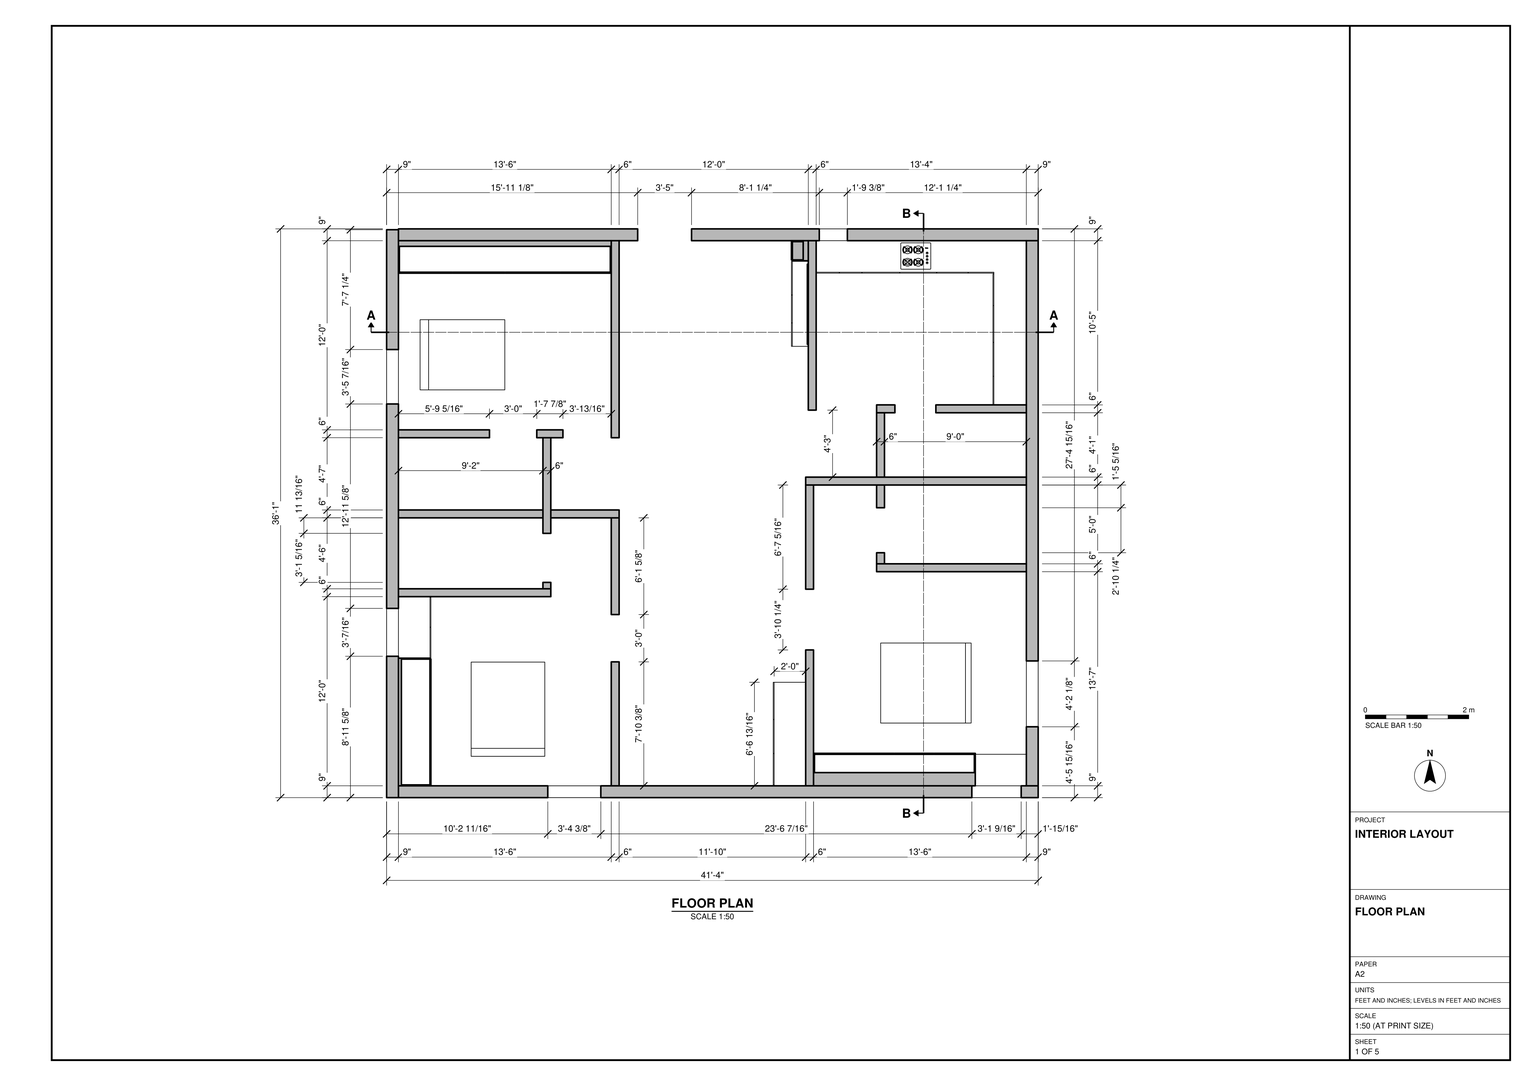
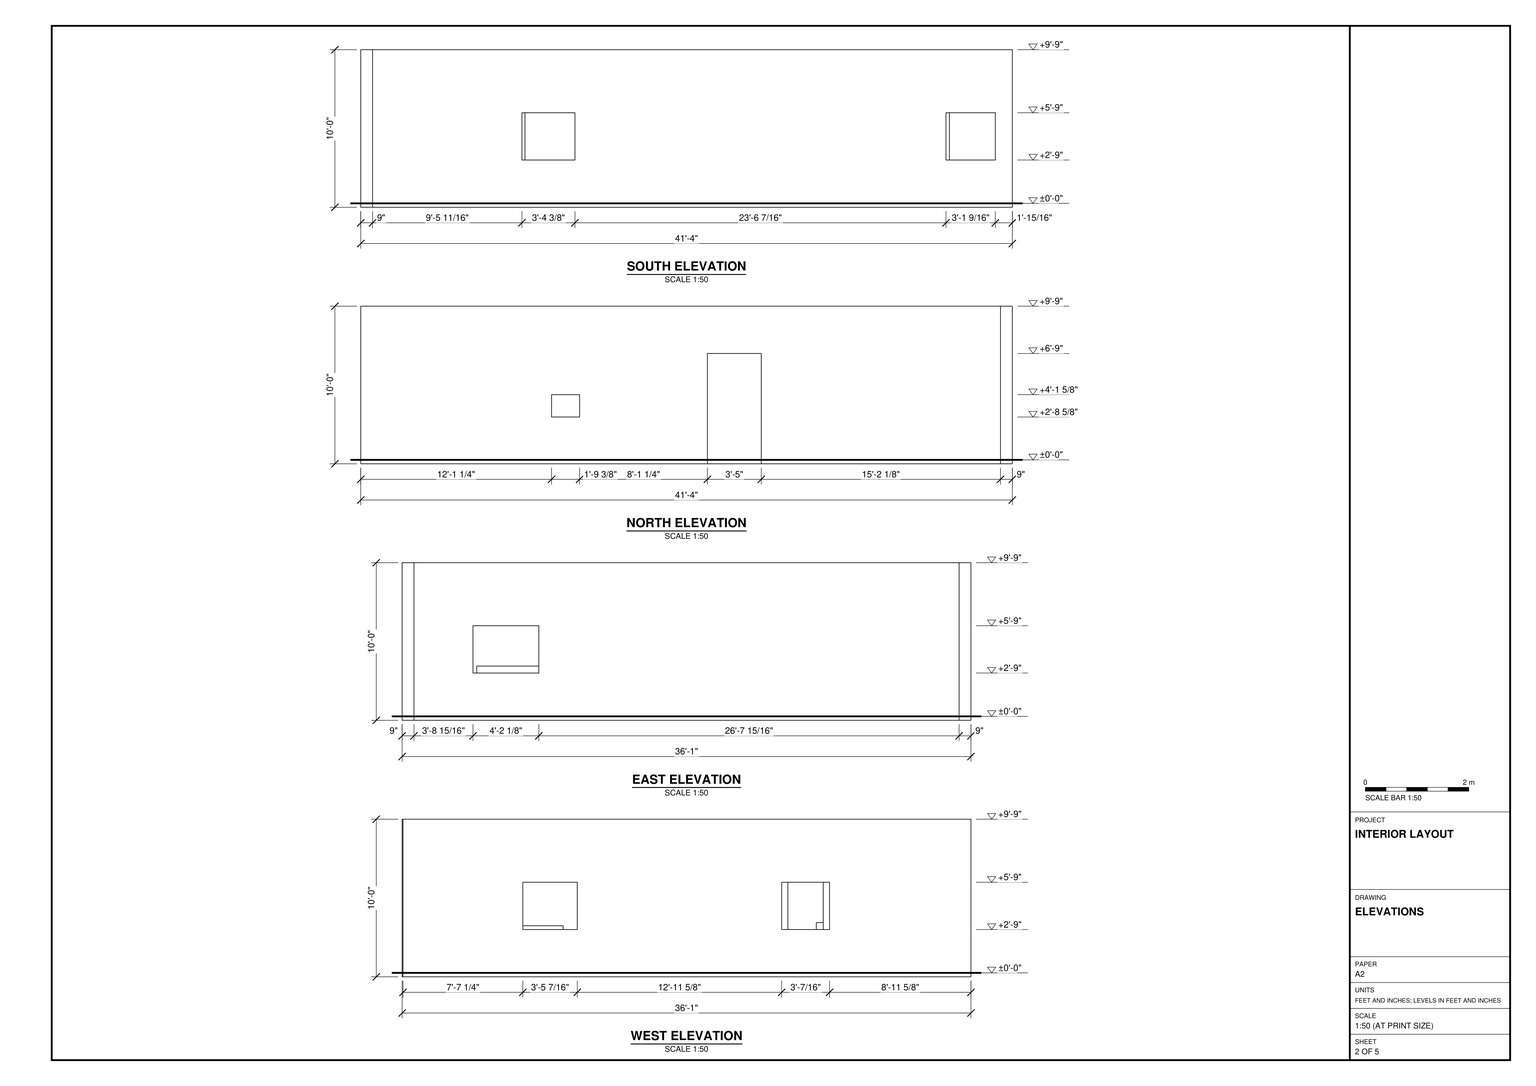
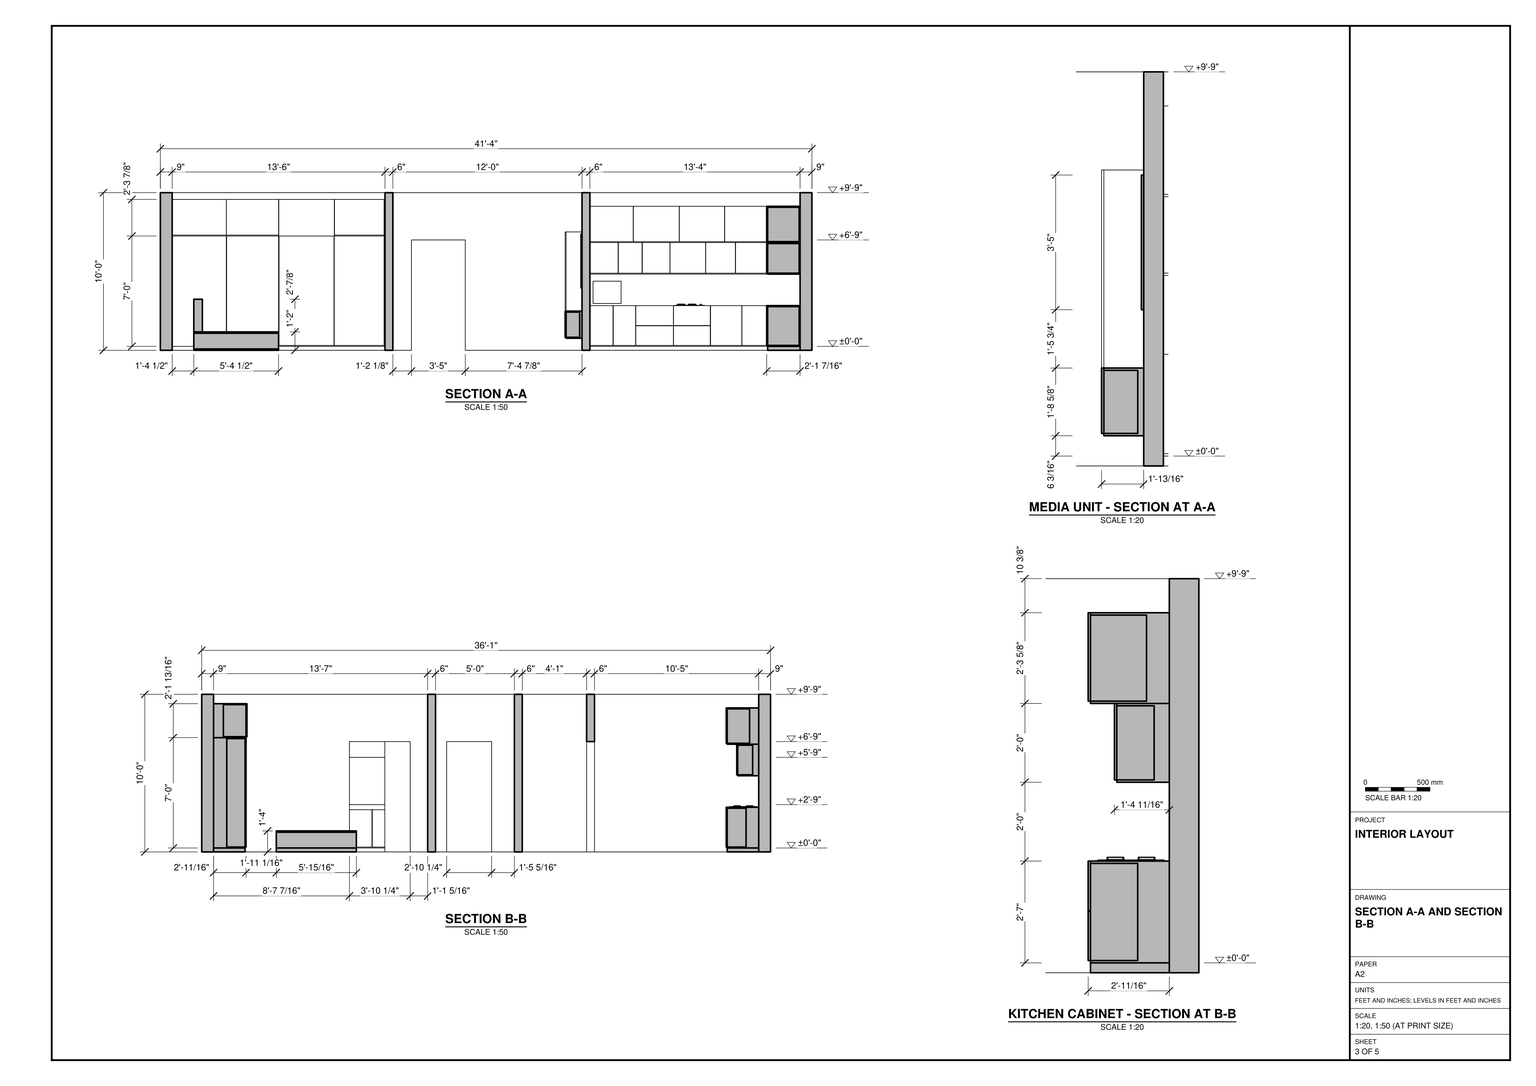
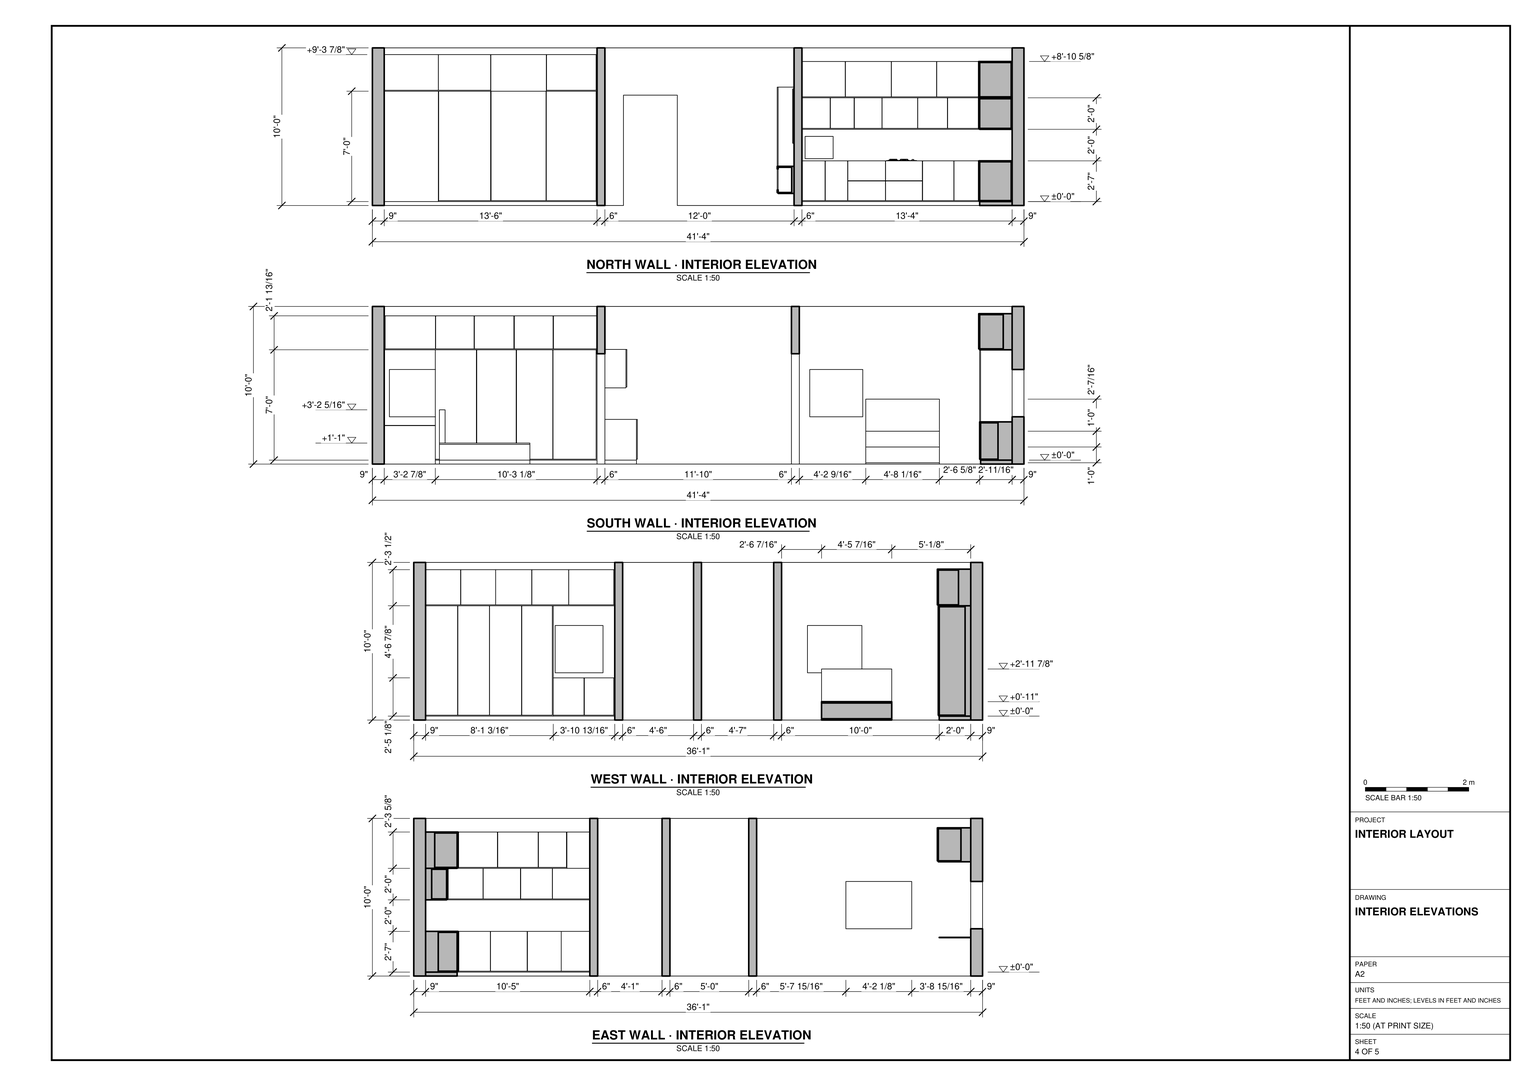
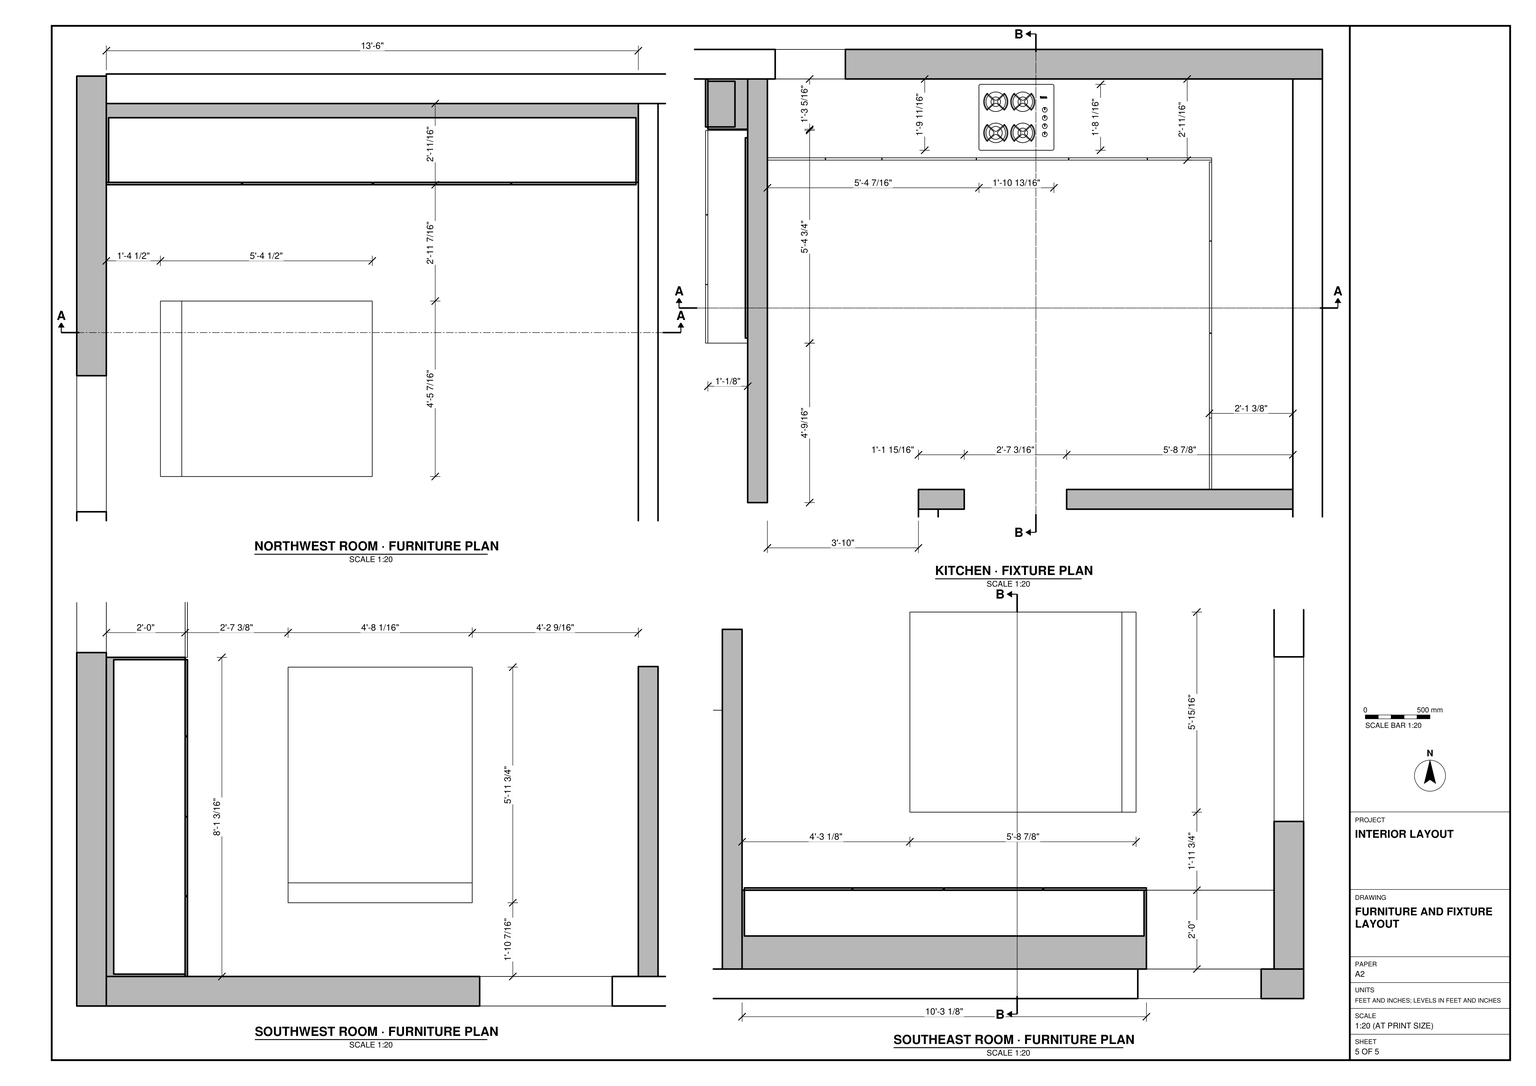
Build the single-storey interior in SketchUp from task_files/diagram_01.pdf. Work in feet and inches. Set the ground-floor datum at ±0'-0" and make the model 41'-4" east to west, 36'-1" north to south and 10'-0" high overall.

Lay out the 9" perimeter walls and 6" internal partitions from the floor plan. Keep the central circulation space open between the bedrooms and kitchen, and follow the partition returns and doorway gaps on either side. Use the elevations to distinguish the floor-level entrance on the north side from the raised window openings and to set the sills and heads.

Fit the northeast kitchen with a counter that turns along the east wall. Use the sections to set the depths and vertical arrangement of the cabinets, and place the cooktop on the north run. On the circulation side of the kitchen partition, model the media unit with its raised lower cabinet. Place the beds and wall storage in the northwest, southwest and southeast rooms, matching their footprints and orientations to the plan. Decor and loose items may be any suitable library components.

Keep shell elements such as walls and slabs separate, make each furniture or joinery piece a group or component, and use components for repeated parts. Save one SketchUp model as output_files/three_bedroom_interior_kitchen_and_built_in_storage.skp.

# SketchUp Ruby script. Lengths in inches.
U = 1.inch
M = Sketchup.active_model
def pt(a) = Geom::Point3d.new(a.map { |v| v * U })
def face(e, loops, mat)
  f = e.add_face(loops[0].map { |a| pt(a) })
  loops[1..].each { |l| e.add_face(l.map { |a| pt(a) }).erase! }
  f.material = f.back_material = mat if mat
  f
end
# faces: each face lists its corners as indices into pts; further lists are holes
def faces(e, pts, list, mat = nil) = list.each { |f| face(e, (f[0].is_a?(Array) ? f : [f]).map { |l| l.map { |i| pts[i] } }, mat) }
# xy, xz, yz: faces in a plane at the given z, y or x. An outline is a flat list of corners, or four numbers for a rectangle; further outlines are holes
def ring(l) = l.size == 4 ? [[l[0], l[1]], [l[2], l[1]], [l[2], l[3]], [l[0], l[3]]] : l.each_slice(2).to_a
def flat(e, list, mat, &to3) = list.each { |f| face(e, (f[0].is_a?(Array) ? f : [f]).map { |l| ring(l).map { |u, v| to3.(u, v) } }, mat) }
def xy(e, z, list, mat = nil) = flat(e, list, mat) { |x, y| [x, y, z] }
def xz(e, y, list, mat = nil) = flat(e, list, mat) { |x, z| [x, y, z] }
def yz(e, x, list, mat = nil) = flat(e, list, mat) { |y, z| [x, y, z] }
def lines(e, pts, list) = list.each { |a, b| e.add_line(pt(pts[a]), pt(pts[b])) }
# prism: a flat outline (further loops are holes) pulled along v
def prism(e, loops, v, mat = nil)
  f = face(e, loops, mat); d = Geom::Vector3d.new(v.map { |x| x * U })
  f.pushpull(f.normal.samedirection?(d) ? d.length : -d.length)
end
def box(e, o, s, mat = nil) = prism(e, [[o, [o[0] + s[0], o[1], o[2]], [o[0] + s[0], o[1] + s[1], o[2]], [o[0], o[1] + s[1], o[2]]]], [0, 0, s[2]], mat)
def at(x, y, z, deg = 0) = Geom::Transformation.translation(pt([x, y, z])) * Geom::Transformation.rotation(ORIGIN, Z_AXIS, deg.degrees)
def axes(o, x, y, z) = Geom::Transformation.new([*x, 0, *y, 0, *z, 0, *pt(o).to_a, 1])
def part(name) = M.definitions.add(name)
# library, detail: a bought-in or finely detailed component or shape, given as its bounding box
def library(name, o, s) = part(name).tap { |d| box(d.entities, o, s) }
def detail(e, o, s) = box(e.add_group.entities, o, s)
def put(e, d, t, mat = nil) = e.add_instance(d, t).tap { |i| i.material = mat if mat }
def group(e, t, mat = nil) = e.add_group.tap { |g| g.transformation = t; g.material = mat if mat }.entities
root = M.entities
c1 = library("1-TABLE DE CUISSON CLC2",[-11.42,-10.04,0],[22.84,20.08,1.26])
c2 = part("Group\#94")
box(c2.entities,[0,0,0],[8.25,13.9,0.71])
put(root,c1,at(402.83,412.33,34))
g1 = group(root,at(0,0,0))
prism(g1,[[[0,432.35,0],[0,0,0],[0,0,120],[0,432.35,120]],[[0,341.125,72],[0,299.6875,72],[0,299.6875,36],[0,341.125,36]],[[0,107.625,72],[0,107.625,36],[0,144.0625,36],[0,144.0625,72]]],[9,0,0])
g2 = group(root,at(9,0,0))
prism(g2,[[[0,0,0],[487,0,0],[487,0,120],[0,0,120]],[[113.6875,0,72],[154.0625,0,72],[154.0625,0,36],[113.6875,0,36]],[[436.5,0,72],[474.0625,0,72],[474.0625,0,36],[436.5,0,36]]],[0,9,0])
g3 = group(root,at(171,9,0))
prism(g3,[[[0,204,0],[0,130.375,0],[0,130.375,84],[0,94.375,84],[0,94.375,0],[0,0,0],[0,0,120],[0,204,120]]],[6,0,0])
g4 = group(root,at(9,153,0))
box(g4,[0,0,0],[116,6,120])
g5 = group(root,at(119,159,0))
xy(g5,0,[[0,0,6,4.875],[0,42.1875,6,115]])
xy(g5,84,[[0,4.875,6,42.1875]])
xy(g5,120,[[0,0,6,115]])
xz(g5,0,[[0,0,6,120]])
xz(g5,4.875,[[0,0,6,84]])
xz(g5,42.1875,[[0,0,6,84]])
xz(g5,115,[[0,0,6,120]])
yz(g5,0,[[0,0,0,120,54,120,54,0,42.1875,0,42.1875,84,4.875,84,4.875,0],[54,0,60,120],[60,0,115,120]])
yz(g5,6,[[0,0,4.875,0,4.875,84,42.1875,84,42.1875,0,54,0,54,120,0,120],[54,0,60,120],[60,0,115,120]])
g6 = group(root,at(9,274,0))
prism(g6,[[[69.3125,6,0],[0,6,0],[0,6,120],[162,6,120],[162,6,84],[125.22,6,84],[125.22,6,0],[105.3125,6,0],[105.3125,6,84],[69.3125,6,84]]],[0,-6,0])
g7 = group(root,at(171,274,0))
prism(g7,[[[0,150,0],[6,150,0],[6,0,0],[0,0,0],[0,141.51,0]]],[0,0,120])
g8 = group(root,at(9,424,0))
prism(g8,[[[182.125,9,0],[0,9,0],[0,9,120],[487,9,120],[487,9,0],[223.125,9,0],[223.125,9,84],[182.125,9,84]],[[320.375,9,52.625],[320.375,9,35.625],[341.75,9,35.625],[341.75,9,52.625]]],[0,-9,0])
g9 = group(root,at(321,295,0))
box(g9,[0,0,0],[6,129,120])
g10 = group(root,at(487,9,0))
prism(g10,[[[0,415,0],[0,0,0],[0,0,120],[0,415,120]],[[0,95.0625,36],[0,95.0625,72],[0,44.9375,72],[0,44.9375,36]]],[9,0,0])
g11 = group(root,at(373,293,0))
prism(g11,[[[13.9375,6,0],[0,6,0],[0,6,120],[114,6,120],[114,6,0],[45.125,6,0],[45.125,6,84],[13.9375,6,84]]],[0,-6,0])
g12 = group(root,at(373,244,0))
box(g12,[0,0,0],[6,49,120])
g13 = group(root,at(319,238,0))
box(g13,[0,0,0],[168,6,120])
g14 = group(root,at(373,172,0))
box(g14,[0,0,0],[114,6,120])
g15 = group(root,at(373,178,0))
prism(g15,[[[6,0,0],[6,8.4375,0],[6,8.4375,84],[6,42.6875,84],[6,42.6875,0],[6,60,0],[6,60,120],[6,0,120]]],[-6,0,0])
g16 = group(root,at(319,9,0))
prism(g16,[[[6,0,0],[6,103.4375,0],[6,103.4375,84],[6,149.6875,84],[6,149.6875,0],[6,229,0],[6,229,120],[6,0,120]]],[-6,0,0])
g17 = group(root,at(125,213,0))
box(g17,[0,0,0],[52,6,120])
g18 = group(root,at(9,213,0))
box(g18,[0,0,0],[110,6,120])
g19 = group(root,at(327,400,0))
prism(g19,[[[0,0,0],[0,24,0],[160,24,0],[160,-101,0],[135.29,-101,0],[135.29,0,0]]],[0,0,3])
g20 = group(root,at(327,299,3))
xy(g20,0,[[135.29,0,135.29,101,0,101,0,125,160,125,160,0]])
xy(g20,0.71,[[135.29,0,159.29,0,159.29,115.375,0.71,115.375,0.71,101,135.29,101]])
xy(g20,30.29,[[135.29,0,135.29,101,0.71,101,0.71,115.375,159.29,115.375,159.29,0]])
xy(g20,31,[[135.29,0,160,0,160,125,0,125,0,101,135.29,101]])
xz(g20,0,[[135.29,0,160,0,160,31,135.29,31,135.29,30.29,159.29,30.29,159.29,0.71,135.29,0.71]])
xz(g20,101,[[0,0,135.29,0,135.29,0.71,0.71,0.71,0.71,30.29,135.29,30.29,135.29,31,0,31]])
xz(g20,115.375,[[0.71,0.71,159.29,30.29]])
xz(g20,125,[[0,0,160,31]])
yz(g20,0,[[101,0,125,31]])
yz(g20,0.71,[[101,0.71,115.375,30.29]])
yz(g20,135.29,[[0,0,101,0.71],[0,30.29,101,31]])
yz(g20,159.29,[[0,0.71,115.375,30.29]])
yz(g20,160,[[0,0,125,31]])
g21 = group(root,at(327,399.29,3.71))
box(g21,[0,0,0],[17.58,0.71,30.29])
g22 = group(root,at(344.78,399.29,3.71))
box(g22,[0,0,0],[17.03,0.71,30.29])
g23 = group(root,at(361.94,399.29,3.71))
prism(g23,[[[0,0.71,30.29],[0,0.71,0],[0,0,0],[0,0,14.95],[0,0.375,14.95],[0,0.375,15.15],[0,0,15.15],[0,0,30.29]]],[28.625,0,0])
g24 = group(root,at(390.68,399.29,3.71))
xy(g24,0,[[0,0,27.94,0.71]])
xy(g24,14.95,[[0,0,27.94,0.71]])
xy(g24,15.15,[[0,0,27.94,0.71]])
xy(g24,30.29,[[0,0,27.94,0.71]])
xz(g24,0,[[0,0,27.94,14.95],[0,15.15,27.94,30.29]])
xz(g24,0.71,[[0,0,27.94,14.95],[0,14.95,27.94,15.15],[0,15.15,27.94,30.29]])
yz(g24,0,[[0,0,0.71,14.95],[0,15.15,0.71,30.29]])
yz(g24,27.94,[[0,0,0.71,14.95],[0,15.15,0.71,30.29]])
g25 = group(root,at(418.86,399.29,3.71))
box(g25,[0,0,0],[23.78,0.71,30.29])
g26 = group(root,at(442.76,399.29,3.71))
box(g26,[0,0,0],[19.53,0.71,30.29])
g27 = group(root,at(461.58,374.71,3.71))
box(g27,[0,0,0],[0.71,23.99,30.29])
g28 = group(root,at(461.58,346.69,3.71))
box(g28,[0,0,0],[0.71,27.89,30.29])
g29 = group(root,at(461.58,320.74,3.71))
box(g29,[0,0,0],[0.71,25.73,30.29])
g30 = group(root,at(461.58,299,3.71))
box(g30,[0,0,0],[0.71,21.74,30.29])
g31 = group(root,at(327,424,58))
xy(g31,0,[[135.29,-125,135.29,-16,0,-16,0,0,160,0,160,-125]])
xy(g31,0.71,[[135.29,-125,159.29,-125,159.29,-4.625,0.71,-4.625,0.71,-16,135.29,-16]])
xy(g31,23.29,[[135.29,-125,135.29,-16,0.71,-16,0.71,-4.625,159.29,-4.625,159.29,-125]])
xy(g31,24,[[135.29,-125,160,-125,160,0,0,0,0,-16,135.29,-16]])
xz(g31,-125,[[135.29,0,160,0,160,24,135.29,24,135.29,23.29,159.29,23.29,159.29,0.71,135.29,0.71]])
xz(g31,-16,[[0,0,135.29,0,135.29,0.71,0.71,0.71,0.71,23.29,135.29,23.29,135.29,24,0,24]])
xz(g31,-4.625,[[0.71,0.71,159.29,23.29]])
xz(g31,0,[[0,0,160,24]])
yz(g31,0,[[-16,0,0,24]])
yz(g31,0.71,[[-16,0.71,-4.625,23.29]])
yz(g31,135.29,[[-125,0,-16,0.71],[-125,23.29,-16,24]])
yz(g31,159.29,[[-125,0.71,-4.625,23.29]])
yz(g31,160,[[-125,0,0,24]])
g32 = group(root,at(327,407.29,58.71))
box(g32,[0,0,0],[21.47,0.71,23.29])
g33 = group(root,at(348.67,407.29,58.71))
box(g33,[0,0,0],[18.03,0.71,23.29])
g34 = group(root,at(366.91,407.29,58.71))
box(g34,[0,0,0],[21.01,0.71,23.29])
g35 = group(root,at(388.02,407.29,58.71))
box(g35,[0,0,0],[27.04,0.71,23.29])
g36 = group(root,at(415.16,407.29,58.71))
box(g36,[0,0,0],[22.56,0.71,23.29])
g37 = group(root,at(437.9,407.29,58.71))
box(g37,[0,0,0],[24.39,0.71,23.29])
g38 = group(root,at(461.58,380.28,58.71))
box(g38,[0,0,0],[0.71,26.5,23.29])
g39 = group(root,at(461.58,351.78,58.71))
box(g39,[0,0,0],[0.71,28.36,23.29])
g40 = group(root,at(461.58,327.52,58.71))
box(g40,[0,0,0],[0.71,24.06,23.29])
g41 = group(root,at(461.58,299,58.71))
box(g41,[0,0,0],[0.71,28.42,23.29])
g42 = group(root,at(327,424,82))
xy(g42,0,[[135.29,-125,135.29,-24,0,-24,0,0,160,0,160,-125]])
xy(g42,0.71,[[135.29,-125,159.29,-125,159.29,-6.9375,0.71,-6.9375,0.71,-24,135.29,-24]])
xy(g42,26.92,[[135.29,-125,135.29,-24,0.71,-24,0.71,-6.9375,159.29,-6.9375,159.29,-125]])
xy(g42,27.625,[[135.29,-125,160,-125,160,0,0,0,0,-24,135.29,-24]])
xz(g42,-125,[[135.29,0,160,0,160,27.625,135.29,27.625,135.29,26.92,159.29,26.92,159.29,0.71,135.29,0.71]])
xz(g42,-24,[[0,0,135.29,0,135.29,0.71,0.71,0.71,0.71,26.92,135.29,26.92,135.29,27.625,0,27.625]])
xz(g42,-6.9375,[[0.71,0.71,159.29,26.92]])
xz(g42,0,[[0,0,160,27.625]])
yz(g42,0,[[-24,0,0,27.625]])
yz(g42,0.71,[[-24,0.71,-6.9375,26.92]])
yz(g42,135.29,[[-125,0,-24,0.71],[-125,26.92,-24,27.625]])
yz(g42,159.29,[[-125,0.71,-6.9375,26.92]])
yz(g42,160,[[-125,0,0,27.625]])
g43 = group(root,at(327,399.29,82.71))
box(g43,[0,0,0],[32.93,0.71,26.92])
g44 = group(root,at(360.1,399.29,82.71))
box(g44,[0,0,0],[34.9,0.71,26.92])
g45 = group(root,at(395.11,399.29,82.71))
box(g45,[0,0,0],[34.375,0.71,26.92])
g46 = group(root,at(429.63,399.29,82.71))
box(g46,[0,0,0],[32.66,0.71,26.92])
g47 = group(root,at(461.58,369.33,82.71))
box(g47,[0,0,0],[0.71,29.58,26.92])
g48 = group(root,at(461.58,338.32,82.71))
box(g48,[0,0,0],[0.71,30.76,26.92])
g49 = group(root,at(461.58,316.76,82.71))
box(g49,[0,0,0],[0.71,21.35,26.92])
g50 = group(root,at(461.58,299,82))
box(g50,[0,0,0],[0.71,17.43,27.625])
g51 = group(root,at(9,400,0))
box(g51,[0,0,0],[162,24,3])
g52 = group(root,at(9,400,3))
xy(g52,0,[[0,0,162,24]])
xy(g52,0.71,[[0.71,0,161.29,19.6875]])
xy(g52,83.29,[[0.71,0,161.29,19.6875]])
xy(g52,84,[[0,0,162,24]])
xz(g52,0,[[[0,0,162,84],[0.71,0.71,161.29,83.29]]])
xz(g52,19.6875,[[0.71,0.71,161.29,83.29]])
xz(g52,24,[[0,0,162,84]])
yz(g52,0,[[0,0,24,84]])
yz(g52,0.71,[[0,0.71,19.6875,83.29]])
yz(g52,161.29,[[0,0.71,19.6875,83.29]])
yz(g52,162,[[0,0,24,84]])
g53 = group(root,at(9,399.29,3))
box(g53,[0,0,0],[41.2,0.71,84])
g54 = group(root,at(50.46,399.29,3.71))
box(g54,[0,0,0],[39.54,0.71,83.29])
g55 = group(root,at(90.35,399.29,3.71))
box(g55,[0,0,0],[41.84,0.71,83.29])
g56 = group(root,at(132.4,399.29,3.71))
box(g56,[0,0,0],[37.89,0.71,83.29])
g57 = group(root,at(9,424,87))
xy(g57,0,[[0,-24.71,162,0]])
xy(g57,0.71,[[0.71,-24.71,161.29,-9.33]])
xy(g57,27.18,[[0.71,-24.71,161.29,-9.33]])
xy(g57,27.88,[[0,-24.71,162,0]])
xz(g57,-24.71,[[[0,0,162,27.88],[0.71,0.71,161.29,27.18]]])
xz(g57,-9.33,[[0.71,0.71,161.29,27.18]])
xz(g57,0,[[0,0,162,27.88]])
yz(g57,0,[[-24.71,0,0,27.88]])
yz(g57,0.71,[[-24.71,0.71,-9.33,27.18]])
yz(g57,161.29,[[-24.71,0.71,-9.33,27.18]])
yz(g57,162,[[-24.71,0,0,27.88]])
g58 = group(root,at(9,398.58,87.71))
box(g58,[0,0,0],[41.19,0.71,27.18])
g59 = group(root,at(50.24,398.58,87.71))
box(g59,[0,0,0],[39.76,0.71,27.18])
g60 = group(root,at(90.18,398.58,87))
box(g60,[0,0,0],[42.22,0.71,27.88])
g61 = group(root,at(132.59,398.58,87.71))
box(g61,[0,0,0],[37.7,0.71,27.18])
g62 = group(root,at(9,9,0))
box(g62,[0,0,0],[24,144,3])
g63 = group(root,at(9,9,3))
xy(g63,0,[[0,0,24,97.17]])
xy(g63,0.71,[[2.25,0.71,24,96.46]])
xy(g63,83.29,[[2.25,0.71,24,96.46]])
xy(g63,84,[[0,0,24,97.17]])
xz(g63,0,[[0,0,24,84]])
xz(g63,0.71,[[2.25,0.71,24,83.29]])
xz(g63,96.46,[[2.25,0.71,24,83.29]])
xz(g63,97.17,[[0,0,24,84]])
yz(g63,0,[[0,0,97.17,84]])
yz(g63,2.25,[[0.71,0.71,96.46,83.29]])
yz(g63,24,[[[0,0,97.17,84],[0.71,0.71,96.46,83.29]]])
g64 = group(root,at(33,9,3.71))
box(g64,[0,0,0],[0.71,24.34,83.29])
g65 = group(root,at(33,33.5625,3.71))
box(g65,[0,0,0],[0.71,24.02,83.29])
g66 = group(root,at(33,57.7,3.71))
box(g66,[0,0,0],[0.71,24.32,83.29])
g67 = group(root,at(33,82.24,3.71))
box(g67,[0,0,0],[0.71,23.22,83.29])
g68 = group(root,at(9,106.17,3))
xy(g68,0,[[0,0,24,46.83]])
xy(g68,0.71,[[10.75,0.71,24,46.12]])
xy(g68,28.42,[[10.75,0.71,24,46.12]])
xy(g68,29.125,[[0,0,24,46.83]])
xz(g68,0,[[0,0,24,29.125]])
xz(g68,0.71,[[10.75,0.71,24,28.42]])
xz(g68,46.12,[[10.75,0.71,24,28.42]])
xz(g68,46.83,[[0,0,24,29.125]])
yz(g68,0,[[0,0,46.83,29.125]])
yz(g68,10.75,[[0.71,0.71,46.12,28.42]])
yz(g68,24,[[[0,0,46.83,29.125],[0.71,0.71,46.12,28.42]]])
g69 = group(root,at(33,106.17,3.71))
box(g69,[0,0,0],[0.71,23.41,28.42])
g70 = group(root,at(33,129.86,3.71))
box(g70,[0,0,0],[0.71,22.43,28.42])
g71 = group(root,at(9,9,87))
xy(g71,0,[[0,0,24.71,144]])
xy(g71,0.71,[[6.77,0.71,24.71,143.29]])
xy(g71,26.78,[[6.77,0.71,24.71,143.29]])
xy(g71,27.49,[[0,0,24.71,144]])
xz(g71,0,[[0,0,24.71,27.49]])
xz(g71,0.71,[[6.77,0.71,24.71,26.78]])
xz(g71,143.29,[[6.77,0.71,24.71,26.78]])
xz(g71,144,[[0,0,24.71,27.49]])
yz(g71,0,[[0,0,144,27.49]])
yz(g71,6.77,[[0.71,0.71,143.29,26.78]])
yz(g71,24.71,[[[0,0,144,27.49],[0.71,0.71,143.29,26.78]]])
g72 = group(root,at(33.71,9,87.71))
box(g72,[0,0,0],[0.71,26.64,26.78])
g73 = group(root,at(33.71,35.81,87.71))
box(g73,[0,0,0],[0.71,26.52,26.78])
g74 = group(root,at(33.71,62.32,87.71))
box(g74,[0,0,0],[0.71,27.45,26.78])
g75 = group(root,at(33.71,89.91,87.71))
box(g75,[0,0,0],[0.71,28,26.78])
g76 = group(root,at(33.71,117.98,87.71))
box(g76,[0,0,0],[0.71,34.31,26.78])
g77 = group(root,at(325,9,0))
xy(g77,0,[[0,0,123.12,24]])
xy(g77,3,[[0,0,123.12,24]])
xy(g77,3.71,[[0.71,10.0625,122.41,24]])
xy(g77,86.29,[[0.71,10.0625,122.41,24]])
xy(g77,87,[[0,0,123.12,24]])
xz(g77,0,[[0,0,123.12,3],[0,3,123.12,87]])
xz(g77,10.0625,[[0.71,3.71,122.41,86.29]])
xz(g77,24,[[0,0,123.12,3],[[0,3,123.12,87],[0.71,3.71,122.41,86.29]]])
yz(g77,0,[[0,0,24,3],[0,3,24,87]])
yz(g77,0.71,[[10.0625,3.71,24,86.29]])
yz(g77,122.41,[[10.0625,3.71,24,86.29]])
yz(g77,123.12,[[0,0,24,3],[0,3,24,87]])
g78 = group(root,at(416.83,33,3.71))
box(g78,[0,0,0],[31.29,0.71,83.29])
g79 = group(root,at(386.56,33,3.71))
box(g79,[0,0,0],[29.98,0.71,83.29])
g80 = group(root,at(358.68,33,3.71))
box(g80,[0,0,0],[27.59,0.71,83.29])
g81 = group(root,at(325.71,33,3.71))
box(g81,[0,0,0],[32.78,0.71,83.29])
g82 = group(root,at(325,9,87))
xy(g82,0,[[0,0,162,24.71]])
xy(g82,0.71,[[0.71,7.46,161.29,24.71]])
xy(g82,25.13,[[0.71,7.46,161.29,24.71]])
xy(g82,25.84,[[0,0,162,24.71]])
xz(g82,0,[[0,0,162,25.84]])
xz(g82,7.46,[[0.71,0.71,161.29,25.13]])
xz(g82,24.71,[[[0,0,162,25.84],[0.71,0.71,161.29,25.13]]])
yz(g82,0,[[0,0,24.71,25.84]])
yz(g82,0.71,[[7.46,0.71,24.71,25.13]])
yz(g82,161.29,[[7.46,0.71,24.71,25.13]])
yz(g82,162,[[0,0,24.71,25.84]])
g83 = group(root,at(325,33.71,87.71))
box(g83,[0,0,0],[33.16,0.71,25.13])
g84 = group(root,at(358.47,33.71,87.71))
box(g84,[0,0,0],[29.47,0.71,25.13])
g85 = group(root,at(388.29,33.71,87.71))
box(g85,[0,0,0],[30.06,0.71,25.13])
g86 = group(root,at(418.61,33.71,87.71))
box(g86,[0,0,0],[29.23,0.71,25.13])
g87 = group(root,at(448.02,33.71,87.71))
box(g87,[0,0,0],[38.27,0.71,25.13])
g88 = group(root,at(448.12,9,29.25))
box(g88,[0,0,0],[38.88,24,0.2])
g89 = group(root,at(321,343.5625,9.1875))
xy(g89,0,[[-12.125,0,0,64.75]])
xy(g89,0.71,[[-12.125,0.71,-1.8125,64.04]])
xy(g89,19.92,[[-12.125,0.71,-1.8125,64.04]])
xy(g89,20.625,[[-12.125,0,0,64.75]])
xz(g89,0,[[-12.125,0,0,20.625]])
xz(g89,0.71,[[-12.125,0.71,-1.8125,19.92]])
xz(g89,64.04,[[-12.125,0.71,-1.8125,19.92]])
xz(g89,64.75,[[-12.125,0,0,20.625]])
yz(g89,-12.125,[[[0,0,64.75,20.625],[0.71,0.71,64.04,19.92]]])
yz(g89,-1.8125,[[0.71,0.71,64.04,19.92]])
yz(g89,0,[[0,0,64.75,20.625]])
g90 = group(root,at(308.17,382.77,9.9))
box(g90,[0,0,0],[0.71,25.55,19.92])
g91 = group(root,at(308.17,361.46,9.9))
prism(g91,[[[0.71,0,19.92],[0.71,0,0],[0.71,21.07,0],[0.71,21.07,19.92]],[[0.71,19.07,2],[0.71,2,2],[0.71,2,17.92],[0.71,19.07,17.92]]],[-0.71,0,0])
g92 = group(root,at(308.17,344.27,9.9))
box(g92,[0,-0.71,0],[0.71,17.79,19.92])
g93 = group(root,at(321,408.6875,11.62))
xy(g93,0,[[-12.125,0,0,15.3125]])
xy(g93,0.71,[[-12.125,0.71,-3.875,14.6]])
xy(g93,77.79,[[-12.125,0.71,-3.875,14.6]])
xy(g93,78.5,[[-12.125,0,0,15.3125]])
xz(g93,0,[[-12.125,0,0,78.5]])
xz(g93,0.71,[[-12.125,0.71,-3.875,77.79]])
xz(g93,14.6,[[-12.125,0.71,-3.875,77.79]])
xz(g93,15.3125,[[-12.125,0,0,78.5]])
yz(g93,-12.125,[[[0,0,15.3125,78.5],[0.71,0.71,14.6,77.79]]])
yz(g93,-3.875,[[0.71,0.71,14.6,77.79]])
yz(g93,0,[[0,0,15.3125,78.5]])
put(root,c2,at(308.875,409.4,31.42))
put(root,c2,at(308.875,409.4,50.52))
put(root,c2,at(308.875,409.4,69.61))
g94 = group(root,at(308.17,409.4,12.33))
box(g94,[0,0,0],[0.71,14.6,77.79])
g95 = group(root,at(321,345.1,47.57))
box(g95,[-0.71,0,0],[0.71,61,41])
g96 = group(root,at(295,9,0))
box(g96,[0,0,0],[24,78.8125,3])
g97 = group(root,at(295,9,3))
xy(g97,0,[[0,0,24,78.8125]])
xy(g97,0.71,[[0,0.71,11.4375,78.1]])
xy(g97,30.29,[[0,0.71,11.4375,78.1]])
xy(g97,31,[[0,0,24,78.8125]])
xz(g97,0,[[0,0,24,31]])
xz(g97,0.71,[[0,0.71,11.4375,30.29]])
xz(g97,78.1,[[0,0.71,11.4375,30.29]])
xz(g97,78.8125,[[0,0,24,31]])
yz(g97,0,[[[0,0,78.8125,31],[0.71,0.71,78.1,30.29]]])
yz(g97,11.4375,[[0.71,0.71,78.1,30.29]])
yz(g97,24,[[0,0,78.8125,31]])
g98 = group(root,at(294.29,59.57,3.71))
box(g98,[0,0,0],[0.71,28.24,30.29])
g99 = group(root,at(294.29,33.69,3.71))
box(g99,[0,0,0],[0.71,25.7,30.29])
g100 = group(root,at(294.29,9.71,3.71))
box(g100,[0,0,0],[0.71,23.83,30.29])
g101 = group(root,at(319,9,58))
xy(g101,0,[[-16,0,0,78.8125]])
xy(g101,0.71,[[-16,0.71,-6.5,78.1]])
xy(g101,28.57,[[-16,0.71,-6.5,78.1]])
xy(g101,29.28,[[-16,0,0,78.8125]])
xz(g101,0,[[-16,0,0,29.28]])
xz(g101,0.71,[[-16,0.71,-6.5,28.57]])
xz(g101,78.1,[[-16,0.71,-6.5,28.57]])
xz(g101,78.8125,[[-16,0,0,29.28]])
yz(g101,-16,[[[0,0,78.8125,29.28],[0.71,0.71,78.1,28.57]]])
yz(g101,-6.5,[[0.71,0.71,78.1,28.57]])
yz(g101,0,[[0,0,78.8125,29.28]])
g102 = group(root,at(302.29,56.61,58.71))
box(g102,[0,0,0],[0.71,31.2,28.57])
g103 = group(root,at(302.29,31.56,58.71))
box(g103,[0,0,0],[0.71,24.9,28.57])
g104 = group(root,at(302.29,9.71,58.71))
box(g104,[0,0,0],[0.71,21.72,28.57])
g105 = group(root,at(376.1,56.77,0))
box(g105,[0,0,0],[68.875,60.9375,3])
g106 = group(root,at(376.1,56.77,3))
box(g106,[0,0,0],[68.875,60.9375,12])
g107 = group(root,at(376.1,56.77,15))
box(g107,[0,0,0],[68.875,60.9375,1])
g108 = group(root,at(440.66,56.77,16))
box(g108,[0,0,0],[4.3125,60.9375,25.3125])
g109 = group(root,at(64.35,31.45,0))
box(g109,[0,0,0],[56.0625,71.75,1])
g110 = group(root,at(64.35,31.45,1))
box(g110,[0,0,0],[56.0625,71.75,12])
g111 = group(root,at(64.35,31.45,13))
box(g111,[0,0,0],[56.0625,71.75,12])
g112 = group(root,at(64.35,31.45,25))
box(g112,[0,0,0],[56.0625,6.0625,24.4375])
g113 = group(root,at(25.48,310.42,0))
box(g113,[0,0,0],[64.5,53.4375,1])
g114 = group(root,at(25.48,310.42,1))
box(g114,[0,0,0],[64.5,53.4375,12])
g115 = group(root,at(25.48,310.42,13))
box(g115,[0,0,0],[64.5,53.4375,1])
g116 = group(root,at(25.48,310.42,14))
box(g116,[0,0,0],[6.5,53.4375,24.875])
